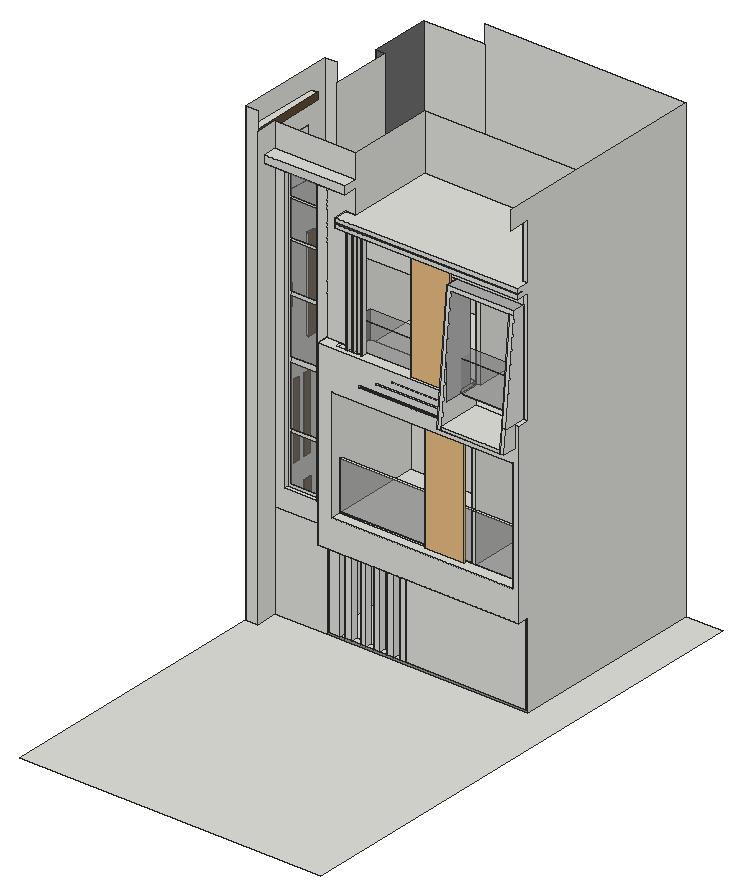
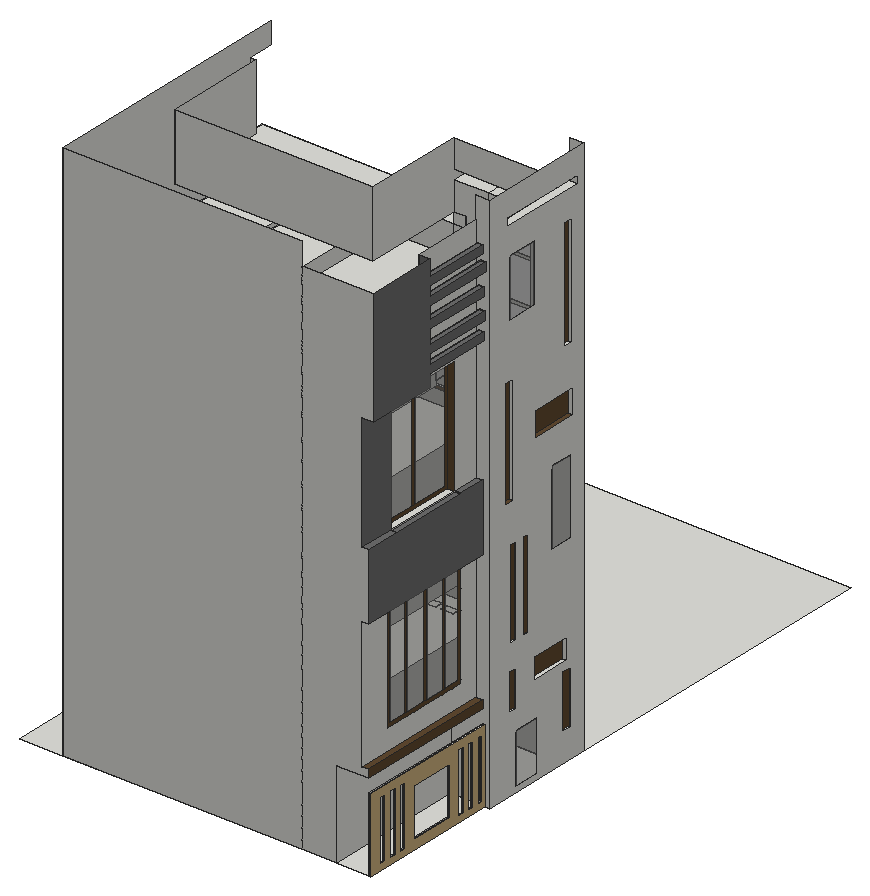
# SketchUp Ruby script. Lengths in inches.
U = 1.inch
M = Sketchup.active_model
def pt(a) = Geom::Point3d.new(a.map { |v| v * U })
def face(e, loops, mat)
  f = e.add_face(loops[0].map { |a| pt(a) })
  loops[1..].each { |l| e.add_face(l.map { |a| pt(a) }).erase! }
  f.material = f.back_material = mat if mat
  f
end
# faces: each face lists its corners as indices into pts; further lists are holes
def faces(e, pts, list, mat = nil) = list.each { |f| face(e, (f[0].is_a?(Array) ? f : [f]).map { |l| l.map { |i| pts[i] } }, mat) }
# xy, xz, yz: faces in a plane at the given z, y or x. An outline is a flat list of corners, or four numbers for a rectangle; further outlines are holes
def ring(l) = l.size == 4 ? [[l[0], l[1]], [l[2], l[1]], [l[2], l[3]], [l[0], l[3]]] : l.each_slice(2).to_a
def flat(e, list, mat, &to3) = list.each { |f| face(e, (f[0].is_a?(Array) ? f : [f]).map { |l| ring(l).map { |u, v| to3.(u, v) } }, mat) }
def xy(e, z, list, mat = nil) = flat(e, list, mat) { |x, y| [x, y, z] }
def xz(e, y, list, mat = nil) = flat(e, list, mat) { |x, z| [x, y, z] }
def yz(e, x, list, mat = nil) = flat(e, list, mat) { |y, z| [x, y, z] }
def lines(e, pts, list) = list.each { |a, b| e.add_line(pt(pts[a]), pt(pts[b])) }
# prism: a flat outline (further loops are holes) pulled along v
def prism(e, loops, v, mat = nil)
  f = face(e, loops, mat); d = Geom::Vector3d.new(v.map { |x| x * U })
  f.pushpull(f.normal.samedirection?(d) ? d.length : -d.length)
end
def box(e, o, s, mat = nil) = prism(e, [[o, [o[0] + s[0], o[1], o[2]], [o[0] + s[0], o[1] + s[1], o[2]], [o[0], o[1] + s[1], o[2]]]], [0, 0, s[2]], mat)
def at(x, y, z, deg = 0) = Geom::Transformation.translation(pt([x, y, z])) * Geom::Transformation.rotation(ORIGIN, Z_AXIS, deg.degrees)
def axes(o, x, y, z) = Geom::Transformation.new([*x, 0, *y, 0, *z, 0, *pt(o).to_a, 1])
def part(name) = M.definitions.add(name)
# library, detail: a bought-in or finely detailed component or shape, given as its bounding box
def library(name, o, s) = part(name).tap { |d| box(d.entities, o, s) }
def detail(e, o, s) = box(e.add_group.entities, o, s)
def put(e, d, t, mat = nil) = e.add_instance(d, t).tap { |i| i.material = mat if mat }
def group(e, t, mat = nil) = e.add_group.tap { |g| g.transformation = t; g.material = mat if mat }.entities
root = M.entities
M.materials.add("Niraj_Hair_Dark").color = [109, 109, 109]
M.materials.add("Niraj_Hair_Gray").color = [178, 178, 178]
M.materials.add("Niraj_Shoe_Sole").color = [96, 73, 48]
M.materials.add("[Concrete Aggregate Smoke]").color = [154, 150, 148]
M.materials.add("[Translucent Glass Gray]").color = [128, 128, 128]
M.materials["[Translucent Glass Gray]"].alpha = 0.5
M.materials.add("[Wood Floor Light]").color = [204, 176, 127]
c1 = library("frame",[0,0,0],[50.17,2.92,33.58])
xy(root,0,[[0,0,2067.625,0,2067.625,3443.8125,1819.6,3443.8125,1819.6,2086.95,80.5,2086.95,80.5,1936.0625,0,1936.0625],[0,1936.0625,80.5,1936.0625,80.5,2086.95,433.875,2086.95,433.875,3443.8125,229.125,3443.8125,229.125,2618.125,0,2618.125],[433.875,2086.95,1819.6,3443.8125],[41.65,2618.125,229.125,3443.8125]])
xy(root,17.93,[[451.8,2086.95,525.86,2086.95,525.86,2130.79,469.67,2130.79,469.67,2174.62,451.8,2174.62],[525.86,2086.95,562.16,2130.79],[562.16,2086.95,605.625,2130.79],[605.625,2086.95,672.57,2130.79],[672.57,2086.95,706.36,2130.79],
  [706.36,2086.95,759.87,2130.79],[759.87,2086.95,800.11,2130.79],[800.11,2086.95,846.69,2130.79],[846.69,2086.95,893.05,2130.79],[893.05,2086.95,940.32,2130.79],
  [940.32,2086.95,975.8,2130.79],[975.8,2086.95,1019.63,2130.79]])
xy(root,33.625,[[29.75,2640.58,41.65,2668.46],[29.75,2707.85,41.65,2738.54],[29.75,2773.125,41.65,2815],[29.75,3197.32,41.65,3236.19],[29.75,3266.57,41.65,3305.44],
  [29.75,3340.94,41.65,3379.82]])
xy(root,54.16,[[29.75,2868.64,41.65,3132.7]])
xy(root,170.13,[[0,2030.54,12.75,2092.92]])
xy(root,334.29,[[29.75,2868.64,41.65,3132.7]])
xy(root,381.4375,[[29.75,2773.125,41.65,2815],[29.75,3197.32,41.65,3236.19],[29.75,3266.57,41.65,3305.44],[29.75,3340.94,41.65,3379.82]])
xy(root,381.76,[[29.75,2640.58,41.65,2668.46],[29.75,2707.85,41.65,2738.54]])
xy(root,427.6875,[[29.75,2618.125,41.65,3443.8125]])
xy(root,437.4375,[[0,2428.72,11.0625,2480.14]])
xy(root,481.07,[[0,2030.54,12.75,2092.92]])
xy(root,505.16,[[43.75,2618.125,229.125,3443.8125]],"Niraj_Shoe_Sole")
xy(root,526.79,[[0,2060.65,28,2300.34]])
xy(root,552.09,[[43.75,2618.125,80.5,3443.8125]],"Niraj_Shoe_Sole")
xy(root,586.82,[[433.875,2008.77,1801.68,2086.95],[1801.68,2008.77,1819.6,2086.95],[451.8,2086.95,451.8,2908.45,1801.68,2908.45,1801.68,2086.95,1019.63,2086.95,1019.63,2130.79,975.8,2130.79,975.8,2086.95,940.32,2086.95,940.32,2130.79,893.05,2130.79,893.05,2086.95,846.69,2086.95,846.69,2130.79,800.11,2130.79,800.11,2086.95,759.87,2086.95,759.87,2130.79,706.36,2130.79,706.36,2086.95,672.57,2086.95,672.57,2130.79,605.625,2130.79,605.625,2086.95,562.16,2086.95,562.16,2130.79,525.86,2130.79,525.86,2086.95],[525.86,2086.95,562.16,2130.79],[605.625,2086.95,672.57,2130.79],
  [706.36,2086.95,759.87,2130.79],[800.11,2086.95,846.69,2130.79],[893.05,2086.95,940.32,2130.79],[975.8,2086.95,1019.63,2130.79]])
xy(root,649.42,[[0,2060.65,28,2300.34]],"Niraj_Shoe_Sole")
xy(root,650.3,[[0,2428.72,11.0625,2480.14]])
xy(root,787.44,[[532.5625,2008.77,1778.69,2008.77,1778.69,2085.53,1315.3125,2085.53,1315.3125,2069.78,532.5625,2069.78],[1222.3,2069.78,1315.3125,2085.53],[532.5625,2085.53,1432.875,2685.39],[1460.625,2085.53,1778.69,2685.39]])
xy(root,794.52,[[0,2341.25,8.4375,2380.32]])
xy(root,796.77,[[0,2428.72,10.1875,2474.59]])
xy(root,797.18,[[145.07,2086.95,369.31,2117.7]])
xy(root,1127.63,[[532.5625,2069.78,1778.69,2085.53]])
xy(root,1307.02,[[0,2341.25,8.4375,2380.32],[0,2428.72,10.1875,2474.59]])
xy(root,1307.05,[[42.6875,2618.125,80.5,3443.8125]],"Niraj_Hair_Dark")
xy(root,1529.14,[[0,2449.3,24.625,2510.3]],"Niraj_Shoe_Sole")
xy(root,1559.19,[[[532.5625,2008.77,532.5625,2685.39,1432.875,2685.39,1432.875,2085.53,1460.625,2085.53,1460.625,2685.39,1778.69,2685.39,1778.69,2008.77],[1170.2,2034.73,1460.83,2040.61]]])
xy(root,1650.63,[[1326.6,1920.58,1787.29,2008.77],[715.35,2008.77,1326.6,2023.58]])
xy(root,1667.38,[[715.35,2008.77,1326.6,2023.58]])
xy(root,1674.8,[[1354,1920.58,1757.58,2215.6875]])
xy(root,1689.64,[[80.5,2772.33,125.6875,3237.39]])
xy(root,1689.64,[[42.6875,2772.33,80.5,3237.39]],"Niraj_Hair_Dark")
xy(root,1693.83,[[42.6875,2618.125,80.5,2772.33],[42.6875,3237.39,80.5,3443.8125]],"Niraj_Hair_Dark")
xy(root,1708.35,[[832.17,2008.77,1326.6,2035.95]])
xy(root,1721.66,[[832.17,2008.77,1326.6,2035.95]])
xy(root,1756.95,[[942.85,2008.77,1326.6,2041.33]])
xy(root,1768.13,[[942.85,2008.77,1326.6,2041.33]])
xy(root,1782.63,[[0,2015.07,28.3125,2292.69]],"Niraj_Shoe_Sole")
xy(root,1798.94,[[1757.58,1935.09,1787.29,2008.77],[1787.29,2008.77,1819.6,2086.95],[1354,2090.8125,1757.58,2090.8125,1757.58,2817.95,1373.97,2817.95,1373.97,2233.45,1345.22,2233.45,1345.22,2817.95,635.4,2817.95,635.4,2215.6875,1354,2215.6875]])
xy(root,1827.75,[[433.875,2008.77,1326.6,2008.77,1326.6,2090.8125,635.4,2090.8125,635.4,2078.39,714.28,2078.39,714.28,2046.08,527.27,2046.08,527.27,2078.39,599.92,2078.39,599.92,2086.95,433.875,2086.95],[527.27,2046.08,547.24,2078.39],[547.24,2046.08,599.92,2078.39],[614.21,2046.08,637.61,2078.39],[652.78,2046.08,672.71,2078.39],
  [683.09,2046.08,702.86,2078.39],[599.92,2078.39,635.4,2086.95],[635.4,2090.8125,1326.6,2090.8125,1326.6,2164.08,1354,2164.08,1354,2215.6875,635.4,2215.6875]])
xy(root,1827.75,[[1326.6,2090.8125,1354,2164.08]],"[Translucent Glass Gray]")
xy(root,1928.26,[[0,2015.07,28.3125,2292.69]],"Niraj_Shoe_Sole")
xy(root,2018.69,[[635.4,2090.8125,1757.58,2215.6875]],"[Translucent Glass Gray]")
xy(root,2162.45,[[0,2449.3,24.625,2510.3]],"Niraj_Shoe_Sole")
xy(root,2167.03,[[0,2025.46,22.6875,2082.21]])
xy(root,2366.7,[[16.25,3030.97,16.25,3443.8125,80.5,3443.8125,80.5,3237.39,125.6875,3237.39,125.6875,3030.97]])
xy(root,2366.7,[[80.5,2772.33,125.6875,3030.97]],"Niraj_Shoe_Sole")
xy(root,2412.4,[[635.4,2086.95,1014.27,2817.95]])
xy(root,2434.7,[[16.25,2638.47,47.11,3030.97]],"Niraj_Hair_Dark")
xy(root,2473.31,[[1354,2001.09,1757.58,2164.08]])
xy(root,2484.63,[[16.25,2638.47,47.11,3030.97]],"Niraj_Hair_Dark")
xy(root,2500.71,[[1014.27,2086.95,1014.27,2817.95,1345.22,2817.95,1345.22,2233.45,1373.97,2233.45,1373.97,2817.95,1757.58,2817.95,1757.58,2164.08,1326.6,2164.08,1326.6,2090.85],[1014.27,2086.95,1326.6,2090.85,1326.6,2086.95],[1326.6,2086.95,1787.29,2164.08]])
xy(root,2500.71,[[1326.6,2003.77,1787.29,2086.95]],"Niraj_Hair_Gray")
xy(root,2539.76,[[16.25,2634.85,47.11,3030.97]],"Niraj_Hair_Dark")
xy(root,2573.63,[[637.61,2046.08,652.78,2078.39]])
xy(root,2573.75,[[702.86,2046.08,714.28,2078.39]])
xy(root,2576.13,[[672.71,2046.08,683.09,2078.39]])
xy(root,2578.69,[[599.92,2046.08,614.21,2078.39]])
xy(root,2585.24,[[566.61,1995.45,635.4,2086.95],[635.4,1995.45,1787.29,2086.95],[1787.29,1995.45,1819.6,2086.95]])
xy(root,2589.69,[[16.25,2634.85,47.11,3030.97]],"Niraj_Hair_Dark")
xy(root,2612.93,[[566.61,1995.45,1819.6,2042.52]],"Niraj_Shoe_Sole")
xy(root,2623.44,[[566.61,1995.45,1819.6,2042.52]],"Niraj_Shoe_Sole")
xy(root,2649.48,[[566.61,1995.45,1819.6,1995.45,1819.6,2086.95,1784.73,2086.95,1784.73,2675.33,635.4,2675.33,635.4,2086.95,566.61,2086.95]])
xy(root,2669.45,[[16.25,2642.1,47.11,3030.97]],"Niraj_Hair_Dark")
xy(root,2719.38,[[16.25,2642.1,47.11,3030.97]],"Niraj_Hair_Dark")
xy(root,2790.01,[[16.25,2626.1,47.11,3030.97]],"Niraj_Hair_Dark")
xy(root,2812.28,[[0,2025.46,22.6875,2082.21]])
xy(root,2815.51,[[80.5,1991.27,80.5,2086.95,145.07,2086.95,145.07,2117.7,369.31,2117.7,369.31,2086.95,433.875,2086.95,433.875,1991.27],[433.875,1991.27,635.4,2086.95]])
xy(root,2839.94,[[16.25,2626.1,47.11,3030.97]],"Niraj_Hair_Dark")
xy(root,2869.21,[[80.5,1991.27,635.4,2086.95]])
xy(root,2892.82,[[16.25,2649.22,47.11,3030.97]],"Niraj_Hair_Dark")
xy(root,2942.76,[[16.25,2649.22,47.11,3030.97]],"Niraj_Hair_Dark")
xy(root,2972.14,[[0,1982.93,49.3125,2495.24]])
xy(root,3020.32,[[0,1982.93,49.3125,2495.24]])
xz(root,1920.58,[[1354,1650.63,1757.58,1674.8]])
xz(root,1936.0625,[[0,0,80.5,3161.9375]])
xz(root,1982.93,[[0,2972.14,49.3125,3020.32]])
xz(root,1991.27,[[80.5,2815.51,635.4,2869.21]])
xz(root,1995.45,[[566.61,2585.24,1819.6,2612.93],[566.61,2623.44,1819.6,2649.48]])
xz(root,2008.77,[[[433.875,586.82,1819.6,586.82,1819.6,1798.94,1787.29,1798.94,1787.29,1650.63,715.35,1650.63,715.35,1667.38,1326.6,1667.38,1326.6,1708.35,832.17,1708.35,832.17,1721.66,1326.6,1721.66,1326.6,1756.95,942.85,1756.95,942.85,1768.13,1326.6,1768.13,1326.6,1827.75,433.875,1827.75],[532.5625,787.44,1778.69,1559.19]],[1326.6,1650.63,1370.22,1667.38]])
xz(root,2015.07,[[0,1782.63,28.3125,1928.26]])
xz(root,2023.58,[[715.35,1650.63,1326.6,1667.38]],"Niraj_Shoe_Sole")
xz(root,2025.46,[[0,2167.03,22.6875,2812.28]])
xz(root,2030.54,[[0,170.13,12.75,481.07]])
xz(root,2035.95,[[832.17,1708.35,1326.6,1721.66]],"Niraj_Shoe_Sole")
xz(root,2041.33,[[942.85,1756.95,1326.6,1768.13]],"Niraj_Shoe_Sole")
xz(root,2042.52,[[566.61,2612.93,1819.6,2623.44]],"Niraj_Shoe_Sole")
xz(root,2046.08,[[599.92,1827.75,614.21,2578.69],[637.61,1827.75,652.78,2573.63],[672.71,1827.75,683.09,2576.13],[702.86,1827.75,714.28,2573.75]])
xz(root,2060.65,[[0,526.79,28,649.42]])
xz(root,2078.39,[[599.92,1827.75,614.21,2578.69],[637.61,1827.75,652.78,2573.63],[672.71,1827.75,683.09,2576.13],[702.86,1827.75,714.28,2573.75]])
xz(root,2082.21,[[0,2167.03,22.6875,2812.28]],"Niraj_Shoe_Sole")
xz(root,2085.53,[[1432.875,787.44,1460.625,1127.63],[1432.875,1127.63,1460.625,1559.19]])
xz(root,2085.53,[[532.5625,787.44,1432.875,1127.63],[1460.625,787.44,1778.69,1127.63]],"[Translucent Glass Gray]")
xz(root,2086.95,[[80.5,0,433.875,658.03],[451.8,17.93,525.86,586.82],[562.16,17.93,605.625,586.82],[672.57,17.93,706.36,586.82],[759.87,17.93,800.11,586.82],
  [846.69,17.93,893.05,586.82],[940.32,17.93,975.8,586.82],[975.8,17.93,1801.68,586.82],[80.5,658.03,433.875,658.03,433.875,2815.51,369.31,2815.51,369.31,797.18,145.07,797.18,145.07,2815.51,80.5,2815.51],[1787.29,1798.94,1819.6,2585.24],
  [433.875,1827.75,635.4,1827.75,635.4,2585.24,566.61,2585.24,566.61,2649.48,635.4,2649.48,635.4,2815.51,433.875,2815.51],[635.4,2412.4,1014.27,2412.4,1014.27,2500.71,1787.29,2500.71,1787.29,2585.24,635.4,2585.24],[566.61,2585.24,635.4,2649.48],[1784.73,2649.48,1819.6,3034.69],[80.5,2869.21,635.4,3034.69]])
xz(root,2086.95,[[433.875,0,1819.6,17.93],[433.875,17.93,451.8,586.82],[1801.68,17.93,1819.6,586.82]],"[Concrete Aggregate Smoke]")
xz(root,2090.8125,[[1354,1798.94,1354,1827.75,635.4,1827.75,635.4,2018.69,1757.58,2018.69,1757.58,1798.94]],"[Translucent Glass Gray]")
xz(root,2092.92,[[0,170.13,12.75,481.07]],"Niraj_Shoe_Sole")
xz(root,2117.7,[[145.07,797.18,369.31,797.18,369.31,2815.51,350.03,2815.51,350.03,816.45,164.34,816.45,164.34,2815.51,145.07,2815.51],[164.34,1134.19,350.03,1156.58],[164.34,1567.92,350.03,1599.48],[164.34,1979.26,350.03,2002.15],[164.34,2315.83,350.03,2333.26],
  [164.34,2574.39,350.03,2588.67]])
xz(root,2117.7,[[164.34,816.45,350.03,1134.19],[164.34,1156.58,350.03,1567.92],[164.34,1599.48,350.03,1979.26],[164.34,2002.15,350.03,2315.83],[164.34,2333.26,350.03,2574.39],
  [164.34,2588.67,350.03,2815.51]],"[Translucent Glass Gray]")
xz(root,2130.79,[[469.67,17.93,525.86,586.82]])
xz(root,2164.08,[[1326.6,1827.75,1326.6,2500.71,1757.58,2500.71,1757.58,2473.31,1354,2473.31,1354,1827.75]])
xz(root,2215.6875,[[635.4,1798.94,1354,1827.75]],"[Translucent Glass Gray]")
xz(root,2233.45,[[1345.22,1798.94,1373.97,2500.71]])
xz(root,2292.69,[[0,1782.63,28.3125,1928.26]],"Niraj_Shoe_Sole")
xz(root,2300.34,[[0,526.79,28,649.42]],"Niraj_Shoe_Sole")
xz(root,2341.25,[[0,794.52,8.4375,1307.02]])
xz(root,2380.32,[[0,794.52,8.4375,1307.02]],"Niraj_Shoe_Sole")
xz(root,2428.72,[[0,437.4375,11.0625,650.3],[0,796.77,10.1875,1307.02]])
xz(root,2449.3,[[0,1529.14,24.625,2162.45]])
xz(root,2474.59,[[0,796.77,10.1875,1307.02]],"Niraj_Shoe_Sole")
xz(root,2480.14,[[0,437.4375,11.0625,650.3]],"Niraj_Shoe_Sole")
xz(root,2495.24,[[0,2972.14,49.3125,3020.32]])
xz(root,2510.3,[[0,1529.14,24.625,2162.45]],"Niraj_Shoe_Sole")
xz(root,2618.125,[[0,0,0,3161.9375,80.5,3161.9375,80.5,1693.83,42.6875,1693.83,42.6875,1307.05,80.5,1307.05,80.5,552.09,43.75,552.09,43.75,505.16,229.125,505.16,229.125,0,41.65,0,41.65,427.6875,29.75,427.6875,29.75,0],[29.75,0,41.65,427.6875]])
xz(root,2626.1,[[16.25,2790.01,47.11,2839.94]],"Niraj_Hair_Dark")
xz(root,2634.85,[[16.25,2539.76,47.11,2589.69]],"Niraj_Hair_Dark")
xz(root,2638.47,[[16.25,2434.7,47.11,2484.63]],"Niraj_Hair_Dark")
xz(root,2640.58,[[29.75,33.625,41.65,381.76]])
xz(root,2642.1,[[16.25,2669.45,47.11,2719.38]],"Niraj_Hair_Dark")
xz(root,2649.22,[[16.25,2892.82,47.11,2942.76]],"Niraj_Hair_Dark")
xz(root,2668.46,[[29.75,33.625,41.65,381.76]])
xz(root,2675.33,[[635.4,2649.48,1784.73,3034.69]])
xz(root,2685.39,[[532.5625,787.44,1432.875,1559.19],[1460.625,787.44,1778.69,1559.19]])
xz(root,2707.85,[[29.75,33.625,41.65,381.76]])
xz(root,2738.54,[[29.75,33.625,41.65,381.76]])
xz(root,2772.33,[[42.6875,1689.64,80.5,1693.83]],"Niraj_Hair_Dark")
xz(root,2772.33,[[80.5,1689.64,125.6875,2366.7]],"Niraj_Shoe_Sole")
xz(root,2773.125,[[29.75,33.625,41.65,381.4375]])
xz(root,2815,[[29.75,33.625,41.65,381.4375]])
xz(root,2817.95,[[635.4,1798.94,1345.22,1798.94,1345.22,2500.71,1014.27,2500.71,1014.27,2412.4,635.4,2412.4],[1373.97,1798.94,1757.58,2500.71]])
xz(root,2868.64,[[29.75,54.16,41.65,334.29]])
xz(root,2908.45,[[451.8,17.93,1801.68,586.82]])
xz(root,3030.97,[[16.25,2366.7,80.5,2366.7,80.5,3034.69,16.25,3034.69,16.25,2942.76,47.11,2942.76,47.11,2892.82,16.25,2892.82,16.25,2839.94,47.11,2839.94,47.11,2790.01,16.25,2790.01,16.25,2719.38,47.11,2719.38,47.11,2669.45,16.25,2669.45,16.25,2589.69,47.11,2589.69,47.11,2539.76,16.25,2539.76,16.25,2484.63,47.11,2484.63,47.11,2434.7,16.25,2434.7]],"Niraj_Hair_Dark")
xz(root,3132.7,[[29.75,54.16,41.65,334.29]])
xz(root,3197.32,[[29.75,33.625,41.65,381.4375]])
xz(root,3236.19,[[29.75,33.625,41.65,381.4375]])
xz(root,3237.39,[[42.6875,1689.64,80.5,1693.83]],"Niraj_Hair_Dark")
xz(root,3237.39,[[80.5,1689.64,125.6875,2366.7]],"Niraj_Shoe_Sole")
xz(root,3266.57,[[29.75,33.625,41.65,381.4375]])
xz(root,3305.44,[[29.75,33.625,41.65,381.4375]])
xz(root,3340.94,[[29.75,33.625,41.65,381.4375]])
xz(root,3379.82,[[29.75,33.625,41.65,381.4375]])
xz(root,3443.8125,[[229.125,0,229.125,505.16,43.75,505.16,43.75,552.09,80.5,552.09,80.5,1307.05,42.6875,1307.05,42.6875,1693.83,80.5,1693.83,80.5,2366.7,16.25,2366.7,16.25,3034.69,433.875,3034.69,433.875,0],[29.75,0,41.65,427.6875],[433.875,0,1819.6,3161.9375]])
yz(root,0,[[[1936.0625,0,2618.125,3161.9375],[2292.69,2476.34,2473.63,2812.28],[2028.42,1150.09,2165.42,1582.59],[2277.1,29.26,2428.72,324.08],[2015.07,1782.63,2292.69,1928.26],[2449.3,1529.14,2510.3,2162.45],[2025.46,2167.03,2082.21,2812.28],[2060.65,526.79,2300.34,649.42],[1982.93,2972.14,2495.24,3020.32],[2428.72,796.77,2474.59,1307.02],[2341.25,794.52,2380.32,1307.02],[2030.54,170.13,2092.92,481.07],[2428.72,437.4375,2480.14,650.3]]])
yz(root,0,[[2277.1,29.26,2428.72,324.08],[2028.42,1150.09,2165.42,1582.59],[2292.69,2476.34,2473.63,2812.28]],"[Translucent Glass Gray]")
yz(root,8.4375,[[2341.25,794.52,2380.32,1307.02]],"Niraj_Shoe_Sole")
yz(root,10.1875,[[2428.72,796.77,2474.59,1307.02]],"Niraj_Shoe_Sole")
yz(root,11.0625,[[2428.72,437.4375,2480.14,650.3]],"Niraj_Shoe_Sole")
yz(root,12.75,[[2030.54,170.13,2092.92,481.07]],"Niraj_Shoe_Sole")
yz(root,16.25,[[3030.97,2366.7,3030.97,2434.7,2638.47,2434.7,2638.47,2484.63,3030.97,2484.63,3030.97,2539.76,2634.85,2539.76,2634.85,2589.69,3030.97,2589.69,3030.97,2669.45,2642.1,2669.45,2642.1,2719.38,3030.97,2719.38,3030.97,2790.01,2626.1,2790.01,2626.1,2839.94,3030.97,2839.94,3030.97,2892.82,2649.22,2892.82,2649.22,2942.76,3030.97,2942.76,3030.97,3034.69,3443.8125,3034.69,3443.8125,2366.7]],"Niraj_Hair_Dark")
yz(root,22.6875,[[2025.46,2167.03,2082.21,2812.28]],"Niraj_Shoe_Sole")
yz(root,24.625,[[2449.3,1529.14,2510.3,2162.45]],"Niraj_Shoe_Sole")
yz(root,28,[[2060.65,526.79,2300.34,649.42]],"Niraj_Shoe_Sole")
yz(root,28.3125,[[2015.07,1782.63,2292.69,1928.26]],"Niraj_Shoe_Sole")
yz(root,29.75,[[[2618.125,0,3443.8125,427.6875],[2868.64,54.16,3132.7,334.29],[2773.125,33.625,2815,381.4375],[3197.32,33.625,3236.19,381.4375],[3266.57,33.625,3305.44,381.4375],[3340.94,33.625,3379.82,381.4375],[2707.85,33.625,2738.54,381.76],[2640.58,33.625,2668.46,381.76]]],"[Wood Floor Light]")
yz(root,41.65,[[[2618.125,0,3443.8125,427.6875],[2868.64,54.16,3132.7,334.29],[2773.125,33.625,2815,381.4375],[3197.32,33.625,3236.19,381.4375],[3266.57,33.625,3305.44,381.4375],[3340.94,33.625,3379.82,381.4375],[2707.85,33.625,2738.54,381.76],[2640.58,33.625,2668.46,381.76]]])
yz(root,42.6875,[[2618.125,1307.05,2618.125,1693.83,2772.33,1693.83,2772.33,1689.64,3237.39,1689.64,3237.39,1693.83,3443.8125,1693.83,3443.8125,1307.05]],"Niraj_Hair_Dark")
yz(root,43.75,[[2618.125,505.16,3443.8125,552.09]],"Niraj_Shoe_Sole")
yz(root,47.11,[[2638.47,2434.7,3030.97,2484.63],[2634.85,2539.76,3030.97,2589.69],[2642.1,2669.45,3030.97,2719.38],[2626.1,2790.01,3030.97,2839.94],[2649.22,2892.82,3030.97,2942.76]],"Niraj_Hair_Dark")
yz(root,49.3125,[[1982.93,2972.14,2495.24,3020.32]],"Niraj_Shoe_Sole")
yz(root,80.5,[[1936.0625,0,2086.95,0,2086.95,2815.51,1991.27,2815.51,1991.27,2869.21,2086.95,2869.21,2086.95,3034.69,1936.0625,3034.69],[2618.125,552.09,2618.125,1307.05,2726.6,1307.05,2726.6,669.74,3267.35,669.74,3267.35,1307.05,3443.8125,1307.05,3443.8125,552.09],[2772.33,1689.64,3237.39,1693.83],[2618.125,1693.83,2618.125,3034.69,3030.97,3034.69,3030.97,2366.7,2772.33,2366.7,2772.33,1693.83]])
yz(root,80.5,[[3237.39,1693.83,3443.8125,2366.7]],"Niraj_Hair_Dark")
yz(root,80.5,[[[2726.6,669.74,3267.35,1307.05],[2748.21,691.35,3245.74,1285.4375]],[2842.05,691.35,2861.38,1285.4375],[2974.54,691.35,2996.98,1285.4375],[3121.36,691.35,3136.73,1285.4375]],"Niraj_Shoe_Sole")
yz(root,80.5,[[2748.21,691.35,2842.05,1285.4375],[2861.38,691.35,2974.54,1285.4375],[2996.98,691.35,3121.36,1285.4375],[3136.73,691.35,3245.74,1285.4375]],"[Translucent Glass Gray]")
yz(root,125.6875,[[[2772.33,1689.64,3237.39,2366.7],[2789.08,1706.38,3220.64,2349.95]],[3004.86,1706.38,3030.97,2349.95]],"Niraj_Shoe_Sole")
yz(root,125.6875,[[2789.08,1706.38,3004.86,2349.95],[3030.97,1706.38,3220.64,2349.95]],"[Translucent Glass Gray]")
yz(root,145.07,[[2086.95,797.18,2117.7,2815.51]])
yz(root,229.125,[[2618.125,0,3443.8125,505.16]])
yz(root,369.31,[[2086.95,797.18,2117.7,1798.94],[2086.95,1798.94,2117.7,2815.51]])
yz(root,433.875,[[2008.77,586.82,2086.95,732.61],[2008.77,732.61,2086.95,1827.75]])
yz(root,451.8,[[2086.95,17.93,2908.45,586.82]])
yz(root,525.86,[[2086.95,17.93,2130.79,586.82]])
yz(root,532.5625,[[2008.77,787.44,2069.78,787.44,2069.78,1127.63,2085.53,1127.63,2085.53,787.44,2685.39,787.44,2685.39,1559.19,2008.77,1559.19]])
yz(root,562.16,[[2086.95,17.93,2130.79,586.82]])
yz(root,566.61,[[1995.45,2585.24,1995.45,2612.93,2042.52,2612.93,2042.52,2623.44,1995.45,2623.44,1995.45,2649.48,2086.95,2649.48,2086.95,2585.24]])
yz(root,599.92,[[2046.08,1827.75,2078.39,2578.69]],"[Wood Floor Light]")
yz(root,605.625,[[2086.95,17.93,2130.79,586.82]])
yz(root,614.21,[[2046.08,1827.75,2078.39,2578.69]])
yz(root,635.4,[[2215.6875,1798.94,2817.95,1798.94,2817.95,2412.4,2086.95,2412.4,2086.95,1827.75,2090.8125,1827.75,2090.8125,2018.69,2215.6875,2018.69],[2086.95,2649.48,2675.33,2649.48,2675.33,3034.69,2086.95,3034.69,2086.95,2869.21,1991.27,2869.21,1991.27,2815.51,2086.95,2815.51]])
yz(root,635.4,[[2090.8125,1827.75,2215.6875,2018.69]],"[Translucent Glass Gray]")
yz(root,637.61,[[2046.08,1827.75,2078.39,2573.63]],"[Wood Floor Light]")
yz(root,652.78,[[2046.08,1827.75,2078.39,2573.63]])
yz(root,672.57,[[2086.95,17.93,2130.79,586.82]])
yz(root,672.71,[[2046.08,1827.75,2078.39,2576.13]],"[Wood Floor Light]")
yz(root,683.09,[[2046.08,1827.75,2078.39,2576.13]])
yz(root,702.86,[[2046.08,1827.75,2078.39,2573.75]],"[Wood Floor Light]")
yz(root,706.36,[[2086.95,17.93,2130.79,586.82]])
yz(root,714.28,[[2046.08,1827.75,2078.39,2573.75]])
yz(root,715.35,[[2008.77,1650.63,2023.58,1667.38]])
yz(root,759.87,[[2086.95,17.93,2130.79,586.82]])
yz(root,800.11,[[2086.95,17.93,2130.79,586.82]])
yz(root,832.17,[[2008.77,1708.35,2035.95,1721.66]])
yz(root,846.69,[[2086.95,17.93,2130.79,586.82]])
yz(root,893.05,[[2086.95,17.93,2130.79,586.82]])
yz(root,940.32,[[2086.95,17.93,2130.79,586.82]])
yz(root,942.85,[[2008.77,1756.95,2041.33,1768.13]])
yz(root,975.8,[[2086.95,17.93,2130.79,586.82]])
yz(root,1014.27,[[2086.95,2412.4,2817.95,2500.71]])
yz(root,1326.6,[[1920.58,1650.63,2003.77,2500.71,2164.08,2500.71,2164.08,1827.75,2008.77,1827.75,2008.77,1768.13,2041.33,1768.13,2041.33,1756.95,2008.77,1756.95,2008.77,1721.66,2035.95,1721.66,2035.95,1708.35,2008.77,1708.35,2008.77,1650.63],[2008.77,1650.63,2023.58,1667.38]])
yz(root,1345.22,[[2233.45,1798.94,2817.95,2500.71]])
yz(root,1354,[[1920.58,1650.63,1920.58,1674.8,1922.94,1674.8],[1922.94,1674.8,2215.6875,1674.8,2215.6875,1798.94,1960.89,1798.94,1960.89,2062.58]])
yz(root,1354,[[1960.89,1798.94,2090.8125,1798.94,2090.8125,1827.75,2164.08,1827.75,2164.08,2473.31,2001.09,2473.31,1960.89,2062.58]],"Niraj_Hair_Gray")
yz(root,1354,[[2090.8125,1798.94,2215.6875,1827.75]],"[Translucent Glass Gray]")
yz(root,1373.97,[[2233.45,1798.94,2817.95,2500.71]])
yz(root,1432.875,[[2085.53,787.44,2685.39,1559.19]])
yz(root,1460.625,[[2085.53,787.44,2685.39,1559.19]])
yz(root,1757.58,[[1920.58,1650.63,1922.94,1674.8,1920.58,1674.8],[1922.94,1674.8,1935.09,1798.94,2215.6875,1798.94,2215.6875,1674.8],[1935.09,1798.94,2001.09,2473.31,2164.08,2473.31,2164.08,2500.71,2215.6875,2500.71,2215.6875,2018.69,2090.8125,2018.69,2090.8125,1798.94],[2090.8125,1798.94,2090.8125,2018.69,2215.6875,2018.69,2215.6875,2500.71,2817.95,2500.71,2817.95,1798.94]])
yz(root,1778.69,[[2008.77,787.44,2008.77,1559.19,2685.39,1559.19,2685.39,787.44,2085.53,787.44,2085.53,1127.63,2069.78,1127.63,2069.78,787.44]])
yz(root,1784.73,[[2086.95,2649.48,2675.33,3034.69]])
yz(root,1787.29,[[1920.58,1650.63,2008.77,1650.63,2008.77,1798.94,1935.09,1798.94],[1935.09,1798.94,2086.95,1798.94,2086.95,2500.71,2003.77,2500.71,2001.09,2473.31],[2086.95,1798.94,2164.08,2500.71]])
yz(root,1801.68,[[2086.95,17.93,2908.45,586.82]])
yz(root,1819.6,[[2086.95,0,3443.8125,0,3443.8125,3161.9375,1936.0625,3161.9375,1936.0625,3034.69,2086.95,3034.69,2086.95,2649.48,1995.45,2649.48,1995.45,2623.44,2042.52,2623.44,2042.52,2612.93,1995.45,2612.93,1995.45,2585.24,2086.95,2585.24,2086.95,1798.94,2008.77,1798.94,2008.77,586.82,2086.95,586.82]])
p = [[1326.6,2003.77,2500.71],[1326.6,1920.58,1650.63],[1354,1920.58,1650.63],[1354,1922.94,1674.8],[1354,1960.89,2062.58],[1354,2001.09,2473.31],
  [1757.58,2001.09,2473.31],[1787.29,2001.09,2473.31],[1787.29,2003.77,2500.71],[1787.29,1920.58,1650.63],[1787.29,1935.09,1798.94],[1757.58,1935.09,1798.94],
  [1757.58,1922.94,1674.8],[1757.58,1920.58,1650.63],[562.16,2130.79,17.93],[562.16,2174.62,17.93],[1332.74,2090.93,2500.71],[1332.74,2090.93,1798.94],
  [1326.6,2090.85,1798.94],[1787.29,2164.08,1798.94],[1757.58,2164.08,1798.94],[1326.6,2090.85,2500.71],[1014.27,2086.95,1798.94],[1326.6,2090.85,1827.75]]
faces(root,p,[[0,1,2,3,4,5,6,7,8],[9,10,11,12,13],[10,7,6,11]])
lines(root,p,[[14,15],[16,17],[17,18],[19,20],[21,16],[18,22],[18,23]])
put(root,c1,axes([1398.26,2058.2,787.44],[0,0,15.8235],[0,3.96372,0],[-7.91175,0,0]),"Niraj_Shoe_Sole")
put(root,c1,axes([1321.15,2032.93,1827.75],[0,0,15.8235],[0,3.96372,0],[-7.91175,0,0]),"Niraj_Shoe_Sole")
